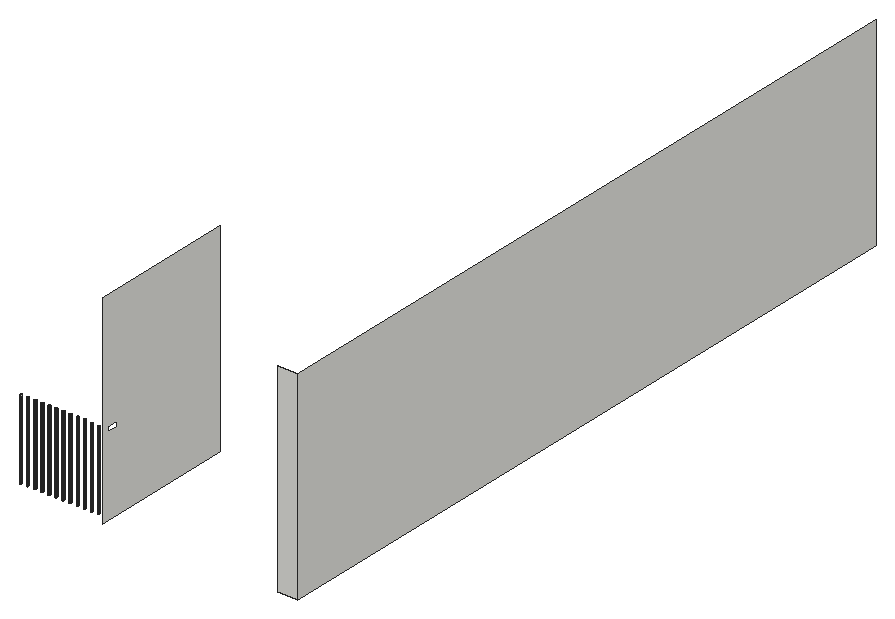
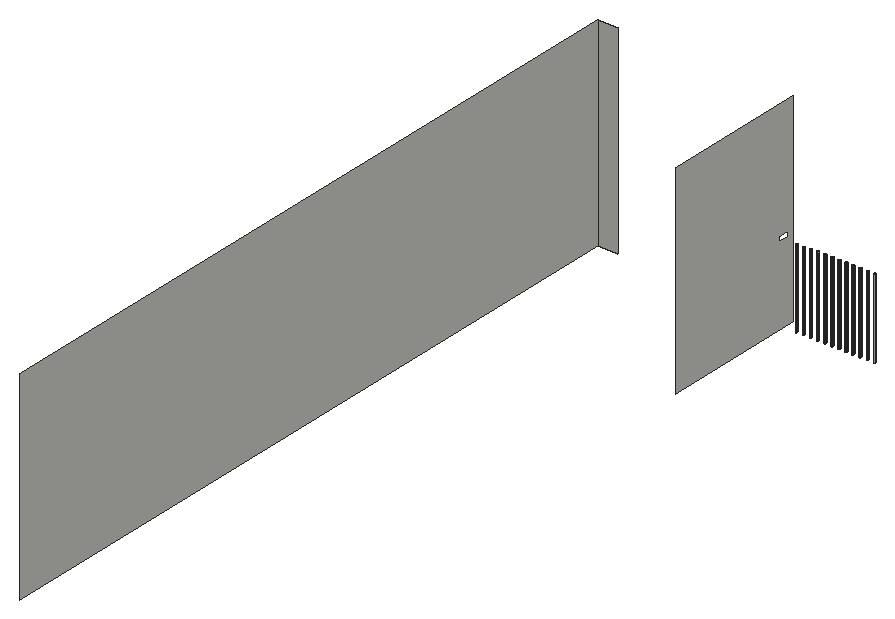
# SketchUp Ruby script. Lengths in inches.
U = 1.inch
M = Sketchup.active_model
def pt(a) = Geom::Point3d.new(a.map { |v| v * U })
def face(e, loops, mat)
  f = e.add_face(loops[0].map { |a| pt(a) })
  loops[1..].each { |l| e.add_face(l.map { |a| pt(a) }).erase! }
  f.material = f.back_material = mat if mat
  f
end
# faces: each face lists its corners as indices into pts; further lists are holes
def faces(e, pts, list, mat = nil) = list.each { |f| face(e, (f[0].is_a?(Array) ? f : [f]).map { |l| l.map { |i| pts[i] } }, mat) }
# xy, xz, yz: faces in a plane at the given z, y or x. An outline is a flat list of corners, or four numbers for a rectangle; further outlines are holes
def ring(l) = l.size == 4 ? [[l[0], l[1]], [l[2], l[1]], [l[2], l[3]], [l[0], l[3]]] : l.each_slice(2).to_a
def flat(e, list, mat, &to3) = list.each { |f| face(e, (f[0].is_a?(Array) ? f : [f]).map { |l| ring(l).map { |u, v| to3.(u, v) } }, mat) }
def xy(e, z, list, mat = nil) = flat(e, list, mat) { |x, y| [x, y, z] }
def xz(e, y, list, mat = nil) = flat(e, list, mat) { |x, z| [x, y, z] }
def yz(e, x, list, mat = nil) = flat(e, list, mat) { |y, z| [x, y, z] }
def lines(e, pts, list) = list.each { |a, b| e.add_line(pt(pts[a]), pt(pts[b])) }
# prism: a flat outline (further loops are holes) pulled along v
def prism(e, loops, v, mat = nil)
  f = face(e, loops, mat); d = Geom::Vector3d.new(v.map { |x| x * U })
  f.pushpull(f.normal.samedirection?(d) ? d.length : -d.length)
end
def box(e, o, s, mat = nil) = prism(e, [[o, [o[0] + s[0], o[1], o[2]], [o[0] + s[0], o[1] + s[1], o[2]], [o[0], o[1] + s[1], o[2]]]], [0, 0, s[2]], mat)
def at(x, y, z, deg = 0) = Geom::Transformation.translation(pt([x, y, z])) * Geom::Transformation.rotation(ORIGIN, Z_AXIS, deg.degrees)
def axes(o, x, y, z) = Geom::Transformation.new([*x, 0, *y, 0, *z, 0, *pt(o).to_a, 1])
def part(name) = M.definitions.add(name)
# library, detail: a bought-in or finely detailed component or shape, given as its bounding box
def library(name, o, s) = part(name).tap { |d| box(d.entities, o, s) }
def detail(e, o, s) = box(e.add_group.entities, o, s)
def put(e, d, t, mat = nil) = e.add_instance(d, t).tap { |i| i.material = mat if mat }
def group(e, t, mat = nil) = e.add_group.tap { |g| g.transformation = t; g.material = mat if mat }.entities
root = M.entities
xy(root,614.8125,[[453.86,132.04,453.64,132.07,453.45,132.15,453.28,132.28,453.15,132.45,453.07,132.64,453.04,132.85,453.07,133.06,453.15,133.26,453.28,133.43,453.45,133.56,453.64,133.64,453.86,133.67,454.07,133.64,454.26,133.56,454.43,133.43,454.56,133.26,454.64,133.06,454.67,132.85,454.64,132.64,454.56,132.45,454.43,132.28,454.26,132.15,454.07,132.07],[459.48,132.04,459.27,132.07,459.07,132.15,458.91,132.28,458.78,132.45,458.7,132.64,458.67,132.85,458.7,133.06,458.78,133.26,458.91,133.43,459.07,133.56,459.27,133.64,459.48,133.67,459.69,133.64,459.89,133.56,460.05,133.43,460.18,133.26,460.27,133.06,460.29,132.85,460.27,132.64,460.18,132.45,460.05,132.28,459.89,132.15,459.69,132.07],[465.54,132.04,465.33,132.07,465.14,132.15,464.97,132.28,464.84,132.45,464.76,132.64,464.73,132.85,464.76,133.06,464.84,133.26,464.97,133.43,465.14,133.56,465.33,133.64,465.54,133.67,465.75,133.64,465.95,133.56,466.12,133.43,466.25,133.26,466.33,133.06,466.36,132.85,466.33,132.64,466.25,132.45,466.12,132.28,465.95,132.15,465.75,132.07],[471.54,132.04,471.33,132.07,471.14,132.15,470.97,132.28,470.84,132.45,470.76,132.64,470.73,132.85,470.76,133.06,470.84,133.26,470.97,133.43,471.14,133.56,471.33,133.64,471.54,133.67,471.75,133.64,471.95,133.56,472.12,133.43,472.25,133.26,472.33,133.06,472.36,132.85,472.33,132.64,472.25,132.45,472.12,132.28,471.95,132.15,471.75,132.07],[477.23,132.04,477.02,132.07,476.82,132.15,476.66,132.28,476.53,132.45,476.45,132.64,476.42,132.85,476.45,133.06,476.53,133.26,476.66,133.43,476.82,133.56,477.02,133.64,477.23,133.67,477.44,133.64,477.64,133.56,477.8,133.43,477.93,133.26,478.02,133.06,478.04,132.85,478.02,132.64,477.93,132.45,477.8,132.28,477.64,132.15,477.44,132.07],
  [483.11,132.04,482.89,132.07,482.7,132.15,482.53,132.28,482.4,132.45,482.32,132.64,482.29,132.85,482.32,133.06,482.4,133.26,482.53,133.43,482.7,133.56,482.89,133.64,483.11,133.67,483.32,133.64,483.51,133.56,483.68,133.43,483.81,133.26,483.89,133.06,483.92,132.85,483.89,132.64,483.81,132.45,483.68,132.28,483.51,132.15,483.32,132.07],[488.98,132.04,488.77,132.07,488.57,132.15,488.41,132.28,488.28,132.45,488.2,132.64,488.17,132.85,488.2,133.06,488.28,133.26,488.41,133.43,488.57,133.56,488.77,133.64,488.98,133.67,489.19,133.64,489.39,133.56,489.55,133.43,489.68,133.26,489.77,133.06,489.79,132.85,489.77,132.64,489.68,132.45,489.55,132.28,489.39,132.15,489.19,132.07],[494.92,132.04,494.71,132.07,494.51,132.15,494.34,132.28,494.21,132.45,494.13,132.64,494.11,132.85,494.13,133.06,494.21,133.26,494.34,133.43,494.51,133.56,494.71,133.64,494.92,133.67,495.13,133.64,495.32,133.56,495.49,133.43,495.62,133.26,495.7,133.06,495.73,132.85,495.7,132.64,495.62,132.45,495.49,132.28,495.32,132.15,495.13,132.07],[500.86,132.04,500.64,132.07,500.45,132.15,500.28,132.28,500.15,132.45,500.07,132.64,500.04,132.85,500.07,133.06,500.15,133.26,500.28,133.43,500.45,133.56,500.64,133.64,500.86,133.67,501.07,133.64,501.26,133.56,501.43,133.43,501.56,133.26,501.64,133.06,501.67,132.85,501.64,132.64,501.56,132.45,501.43,132.28,501.26,132.15,501.07,132.07],[506.67,132.04,506.46,132.07,506.26,132.15,506.09,132.28,505.96,132.45,505.88,132.64,505.86,132.85,505.88,133.06,505.96,133.26,506.09,133.43,506.26,133.56,506.46,133.64,506.67,133.67,506.88,133.64,507.07,133.56,507.24,133.43,507.37,133.26,507.45,133.06,507.48,132.85,507.45,132.64,507.37,132.45,507.24,132.28,507.07,132.15,506.88,132.07],
  [512.54,132.04,512.33,132.07,512.14,132.15,511.97,132.28,511.84,132.45,511.76,132.64,511.73,132.85,511.76,133.06,511.84,133.26,511.97,133.43,512.14,133.56,512.33,133.64,512.54,133.67,512.75,133.64,512.95,133.56,513.12,133.43,513.25,133.26,513.33,133.06,513.36,132.85,513.33,132.64,513.25,132.45,513.12,132.28,512.95,132.15,512.75,132.07],[518.54,132.04,518.33,132.07,518.14,132.15,517.97,132.28,517.84,132.45,517.76,132.64,517.73,132.85,517.76,133.06,517.84,133.26,517.97,133.43,518.14,133.56,518.33,133.64,518.54,133.67,518.75,133.64,518.95,133.56,519.12,133.43,519.25,133.26,519.33,133.06,519.36,132.85,519.33,132.64,519.25,132.45,519.12,132.28,518.95,132.15,518.75,132.07]])
xz(root,124.5,[[673.48,614.8125,690.4375,782.8125]])
yz(root,528.75,[[[124.5,614.8125,246,782.8125],[129.43,680.58,138.74,684.77]]])
yz(root,690.4375,[[124.5,614.8125,724.5,782.8125]])
p = [[453.64,132.07,614.8125],[453.86,132.04,614.8125],[453.86,132.04,680.58],[453.64,132.07,680.58],[454.07,132.07,614.8125],[454.07,132.07,680.58],
  [459.27,132.07,614.8125],[459.48,132.04,614.8125],[459.48,132.04,680.58],[459.27,132.07,680.58],[459.69,132.07,614.8125],[459.69,132.07,680.58],
  [465.33,132.07,614.8125],[465.54,132.04,614.8125],[465.54,132.04,680.58],[465.33,132.07,680.58],[465.75,132.07,614.8125],[465.75,132.07,680.58],
  [471.33,132.07,614.8125],[471.54,132.04,614.8125],[471.54,132.04,680.58],[471.33,132.07,680.58],[471.75,132.07,614.8125],[471.75,132.07,680.58],
  [477.02,132.07,614.8125],[477.23,132.04,614.8125],[477.23,132.04,680.58],[477.02,132.07,680.58],[477.44,132.07,614.8125],[477.44,132.07,680.58],
  [482.89,132.07,614.8125],[483.11,132.04,614.8125],[483.11,132.04,680.58],[482.89,132.07,680.58],[483.32,132.07,614.8125],[483.32,132.07,680.58],
  [488.77,132.07,614.8125],[488.98,132.04,614.8125],[488.98,132.04,680.58],[488.77,132.07,680.58],[489.19,132.07,614.8125],[489.19,132.07,680.58],
  [494.71,132.07,614.8125],[494.92,132.04,614.8125],[494.92,132.04,680.58],[494.71,132.07,680.58],[495.13,132.07,614.8125],[495.13,132.07,680.58],
  [500.64,132.07,614.8125],[500.86,132.04,614.8125],[500.86,132.04,680.58],[500.64,132.07,680.58],[501.07,132.07,614.8125],[501.07,132.07,680.58],
  [506.46,132.07,614.8125],[506.67,132.04,614.8125],[506.67,132.04,680.58],[506.46,132.07,680.58],[506.88,132.07,614.8125],[506.88,132.07,680.58],
  [512.33,132.07,614.8125],[512.54,132.04,614.8125],[512.54,132.04,679.96],[512.33,132.07,679.96],[512.75,132.07,614.8125],[512.75,132.07,679.96],
  [518.33,132.07,614.8125],[518.54,132.04,614.8125],[518.54,132.04,679.96],[518.33,132.07,679.96],[518.75,132.07,614.8125],[518.75,132.07,679.96],
  [453.45,132.15,614.8125],[453.45,132.15,680.58],[454.26,132.15,614.8125],[454.26,132.15,680.58],[459.07,132.15,614.8125],[459.07,132.15,680.58],
  [459.89,132.15,614.8125],[459.89,132.15,680.58],[465.14,132.15,614.8125],[465.14,132.15,680.58],[465.95,132.15,614.8125],[465.95,132.15,680.58],
  [471.14,132.15,614.8125],[471.14,132.15,680.58],[471.95,132.15,614.8125],[471.95,132.15,680.58],[476.82,132.15,614.8125],[476.82,132.15,680.58],
  [477.64,132.15,614.8125],[477.64,132.15,680.58],[482.7,132.15,614.8125],[482.7,132.15,680.58],[483.51,132.15,614.8125],[483.51,132.15,680.58],
  [488.57,132.15,614.8125],[488.57,132.15,680.58],[489.39,132.15,614.8125],[489.39,132.15,680.58],[494.51,132.15,614.8125],[494.51,132.15,680.58],
  [495.32,132.15,614.8125],[495.32,132.15,680.58],[500.45,132.15,614.8125],[500.45,132.15,680.58],[501.26,132.15,614.8125],[501.26,132.15,680.58],
  [506.26,132.15,614.8125],[506.26,132.15,680.58],[507.07,132.15,614.8125],[507.07,132.15,680.58],[512.14,132.15,614.8125],[512.14,132.15,679.96],
  [512.95,132.15,614.8125],[512.95,132.15,679.96],[518.14,132.15,614.8125],[518.14,132.15,679.96],[518.95,132.15,614.8125],[518.95,132.15,679.96],
  [454.43,132.28,614.8125],[454.43,132.28,680.58],[458.91,132.28,614.8125],[458.91,132.28,680.58],[460.05,132.28,614.8125],[460.05,132.28,680.58],
  [464.97,132.28,614.8125],[464.97,132.28,680.58],[466.12,132.28,614.8125],[466.12,132.28,680.58],[470.97,132.28,614.8125],[470.97,132.28,680.58],
  [472.12,132.28,614.8125],[472.12,132.28,680.58],[476.66,132.28,614.8125],[476.66,132.28,680.58],[477.8,132.28,614.8125],[477.8,132.28,680.58],
  [482.53,132.28,614.8125],[482.53,132.28,680.58],[483.68,132.28,614.8125],[483.68,132.28,680.58],[488.41,132.28,614.8125],[488.41,132.28,680.58],
  [489.55,132.28,614.8125],[489.55,132.28,680.58],[494.34,132.28,614.8125],[494.34,132.28,680.58],[495.49,132.28,614.8125],[495.49,132.28,680.58],
  [500.28,132.28,614.8125],[500.28,132.28,680.58],[501.43,132.28,614.8125],[501.43,132.28,680.58],[506.09,132.28,614.8125],[506.09,132.28,680.58],
  [507.24,132.28,614.8125],[507.24,132.28,680.58],[511.97,132.28,614.8125],[511.97,132.28,679.96],[513.12,132.28,614.8125],[513.12,132.28,679.96],
  [517.97,132.28,614.8125],[517.97,132.28,679.96],[519.12,132.28,614.8125],[519.12,132.28,679.96],[454.56,132.45,614.8125],[454.56,132.45,680.58],
  [458.78,132.45,614.8125],[458.78,132.45,680.58],[460.18,132.45,614.8125],[460.18,132.45,680.58],[464.84,132.45,614.8125],[464.84,132.45,680.58],
  [466.25,132.45,614.8125],[466.25,132.45,680.58],[470.84,132.45,614.8125],[470.84,132.45,680.58],[472.25,132.45,614.8125],[472.25,132.45,680.58],
  [476.53,132.45,614.8125],[476.53,132.45,680.58],[477.93,132.45,614.8125],[477.93,132.45,680.58],[482.4,132.45,614.8125],[482.4,132.45,680.58],
  [483.81,132.45,614.8125],[483.81,132.45,680.58],[488.28,132.45,614.8125],[488.28,132.45,680.58],[489.68,132.45,614.8125],[489.68,132.45,680.58],
  [494.21,132.45,614.8125],[494.21,132.45,680.58],[495.62,132.45,614.8125],[495.62,132.45,680.58],[500.15,132.45,614.8125],[500.15,132.45,680.58],
  [501.56,132.45,614.8125],[501.56,132.45,680.58],[505.96,132.45,614.8125],[505.96,132.45,680.58],[507.37,132.45,614.8125],[507.37,132.45,680.58],
  [511.84,132.45,614.8125],[511.84,132.45,679.96],[513.25,132.45,614.8125],[513.25,132.45,679.96],[517.84,132.45,614.8125],[517.84,132.45,679.96],
  [519.25,132.45,614.8125],[519.25,132.45,679.96],[454.64,132.64,614.8125],[454.64,132.64,680.58],[458.7,132.64,614.8125],[458.7,132.64,680.58],
  [460.27,132.64,614.8125],[460.27,132.64,680.58],[464.76,132.64,614.8125],[464.76,132.64,680.58],[466.33,132.64,614.8125],[466.33,132.64,680.58],
  [470.76,132.64,614.8125],[470.76,132.64,680.58],[472.33,132.64,614.8125],[472.33,132.64,680.58],[476.45,132.64,614.8125],[476.45,132.64,680.58],
  [478.02,132.64,614.8125],[478.02,132.64,680.58],[482.32,132.64,614.8125],[482.32,132.64,680.58],[483.89,132.64,614.8125],[483.89,132.64,680.58],
  [488.2,132.64,614.8125],[488.2,132.64,680.58],[489.77,132.64,614.8125],[489.77,132.64,680.58],[494.13,132.64,614.8125],[494.13,132.64,680.58],
  [495.7,132.64,614.8125],[495.7,132.64,680.58],[500.07,132.64,614.8125],[500.07,132.64,680.58],[501.64,132.64,614.8125],[501.64,132.64,680.58],
  [505.88,132.64,614.8125],[505.88,132.64,680.58],[507.45,132.64,614.8125],[507.45,132.64,680.58],[511.76,132.64,614.8125],[511.76,132.64,679.96],
  [513.33,132.64,614.8125],[513.33,132.64,679.96],[517.76,132.64,614.8125],[517.76,132.64,679.96],[519.33,132.64,614.8125],[519.33,132.64,679.96],
  [454.67,132.85,614.8125],[454.67,132.85,680.58],[458.67,132.85,614.8125],[458.67,132.85,680.58],[460.29,132.85,614.8125],[460.29,132.85,680.58],
  [464.73,132.85,614.8125],[464.73,132.85,680.58],[466.36,132.85,614.8125],[466.36,132.85,680.58],[470.73,132.85,614.8125],[470.73,132.85,680.58],
  [472.36,132.85,614.8125],[472.36,132.85,680.58],[476.42,132.85,614.8125],[476.42,132.85,680.58],[478.04,132.85,614.8125],[478.04,132.85,680.58],
  [482.29,132.85,614.8125],[482.29,132.85,680.58],[483.92,132.85,614.8125],[483.92,132.85,680.58],[488.17,132.85,614.8125],[488.17,132.85,680.58],
  [489.79,132.85,614.8125],[489.79,132.85,680.58],[494.11,132.85,614.8125],[494.11,132.85,680.58],[495.73,132.85,614.8125],[495.73,132.85,680.58],
  [500.04,132.85,614.8125],[500.04,132.85,680.58],[501.67,132.85,614.8125],[501.67,132.85,680.58],[505.86,132.85,614.8125],[505.86,132.85,680.58],
  [507.48,132.85,614.8125],[507.48,132.85,680.58],[511.73,132.85,614.8125],[511.73,132.85,679.96],[513.36,132.85,614.8125],[513.36,132.85,679.96],
  [517.73,132.85,614.8125],[517.73,132.85,679.96],[519.36,132.85,614.8125],[519.36,132.85,679.96],[454.64,133.06,614.8125],[454.64,133.06,680.58],
  [458.7,133.06,614.8125],[458.7,133.06,680.58],[460.27,133.06,614.8125],[460.27,133.06,680.58],[464.76,133.06,614.8125],[464.76,133.06,680.58],
  [466.33,133.06,614.8125],[466.33,133.06,680.58],[470.76,133.06,614.8125],[470.76,133.06,680.58],[472.33,133.06,614.8125],[472.33,133.06,680.58],
  [476.45,133.06,614.8125],[476.45,133.06,680.58],[478.02,133.06,614.8125],[478.02,133.06,680.58],[482.32,133.06,614.8125],[482.32,133.06,680.58],
  [483.89,133.06,614.8125],[483.89,133.06,680.58],[488.2,133.06,614.8125],[488.2,133.06,680.58],[489.77,133.06,614.8125],[489.77,133.06,680.58],
  [494.13,133.06,614.8125],[494.13,133.06,680.58],[495.7,133.06,614.8125],[495.7,133.06,680.58],[500.07,133.06,614.8125],[500.07,133.06,680.58],
  [501.64,133.06,614.8125],[501.64,133.06,680.58],[505.88,133.06,614.8125],[505.88,133.06,680.58],[507.45,133.06,614.8125],[507.45,133.06,680.58],
  [511.76,133.06,614.8125],[511.76,133.06,679.96],[513.33,133.06,614.8125],[513.33,133.06,679.96],[517.76,133.06,614.8125],[517.76,133.06,679.96],
  [519.33,133.06,614.8125],[519.33,133.06,679.96],[454.56,133.26,614.8125],[454.56,133.26,680.58],[458.78,133.26,614.8125],[458.78,133.26,680.58],
  [460.18,133.26,614.8125],[460.18,133.26,680.58],[464.84,133.26,614.8125],[464.84,133.26,680.58],[466.25,133.26,614.8125],[466.25,133.26,680.58],
  [470.84,133.26,614.8125],[470.84,133.26,680.58],[472.25,133.26,614.8125],[472.25,133.26,680.58],[476.53,133.26,614.8125],[476.53,133.26,680.58],
  [477.93,133.26,614.8125],[477.93,133.26,680.58],[482.4,133.26,614.8125],[482.4,133.26,680.58],[483.81,133.26,614.8125],[483.81,133.26,680.58],
  [488.28,133.26,614.8125],[488.28,133.26,680.58],[489.68,133.26,614.8125],[489.68,133.26,680.58],[494.21,133.26,614.8125],[494.21,133.26,680.58],
  [495.62,133.26,614.8125],[495.62,133.26,680.58],[500.15,133.26,614.8125],[500.15,133.26,680.58],[501.56,133.26,614.8125],[501.56,133.26,680.58],
  [505.96,133.26,614.8125],[505.96,133.26,680.58],[507.37,133.26,614.8125],[507.37,133.26,680.58],[511.84,133.26,614.8125],[511.84,133.26,679.96],
  [513.25,133.26,614.8125],[513.25,133.26,679.96],[517.84,133.26,614.8125],[517.84,133.26,679.96],[519.25,133.26,614.8125],[519.25,133.26,679.96],
  [454.43,133.43,614.8125],[454.43,133.43,680.58],[458.91,133.43,614.8125],[458.91,133.43,680.58],[460.05,133.43,614.8125],[460.05,133.43,680.58],
  [464.97,133.43,614.8125],[464.97,133.43,680.58],[466.12,133.43,614.8125],[466.12,133.43,680.58],[470.97,133.43,614.8125],[470.97,133.43,680.58],
  [472.12,133.43,614.8125],[472.12,133.43,680.58],[476.66,133.43,614.8125],[476.66,133.43,680.58],[477.8,133.43,614.8125],[477.8,133.43,680.58],
  [482.53,133.43,614.8125],[482.53,133.43,680.58],[483.68,133.43,614.8125],[483.68,133.43,680.58],[488.41,133.43,614.8125],[488.41,133.43,680.58],
  [489.55,133.43,614.8125],[489.55,133.43,680.58],[494.34,133.43,614.8125],[494.34,133.43,680.58],[495.49,133.43,614.8125],[495.49,133.43,680.58],
  [500.28,133.43,614.8125],[500.28,133.43,680.58],[501.43,133.43,614.8125],[501.43,133.43,680.58],[506.09,133.43,614.8125],[506.09,133.43,680.58],
  [507.24,133.43,614.8125],[507.24,133.43,680.58],[511.97,133.43,614.8125],[511.97,133.43,679.96],[513.12,133.43,614.8125],[513.12,133.43,679.96],
  [517.97,133.43,614.8125],[517.97,133.43,679.96],[519.12,133.43,614.8125],[519.12,133.43,679.96],[454.26,133.56,614.8125],[454.26,133.56,680.58],
  [459.07,133.56,614.8125],[459.07,133.56,680.58],[459.89,133.56,614.8125],[459.89,133.56,680.58],[465.14,133.56,614.8125],[465.14,133.56,680.58],
  [465.95,133.56,614.8125],[465.95,133.56,680.58],[471.14,133.56,614.8125],[471.14,133.56,680.58],[471.95,133.56,614.8125],[471.95,133.56,680.58],
  [476.82,133.56,614.8125],[476.82,133.56,680.58],[477.64,133.56,614.8125],[477.64,133.56,680.58],[482.7,133.56,614.8125],[482.7,133.56,680.58],
  [483.51,133.56,614.8125],[483.51,133.56,680.58],[488.57,133.56,614.8125],[488.57,133.56,680.58],[489.39,133.56,614.8125],[489.39,133.56,680.58],
  [494.51,133.56,614.8125],[494.51,133.56,680.58],[495.32,133.56,614.8125],[495.32,133.56,680.58],[500.45,133.56,614.8125],[500.45,133.56,680.58],
  [501.26,133.56,614.8125],[501.26,133.56,680.58],[506.26,133.56,614.8125],[506.26,133.56,680.58],[507.07,133.56,614.8125],[507.07,133.56,680.58],
  [512.14,133.56,614.8125],[512.14,133.56,679.96],[512.95,133.56,614.8125],[512.95,133.56,679.96],[518.14,133.56,614.8125],[518.14,133.56,679.96],
  [518.95,133.56,614.8125],[518.95,133.56,679.96],[453.64,133.64,614.8125],[453.45,133.56,614.8125],[453.45,133.56,680.58],[453.64,133.64,680.58],
  [453.86,133.67,614.8125],[453.86,133.67,680.58],[454.07,133.64,614.8125],[454.07,133.64,680.58],[459.27,133.64,614.8125],[459.27,133.64,680.58],
  [459.48,133.67,614.8125],[459.48,133.67,680.58],[459.69,133.64,614.8125],[459.69,133.64,680.58],[465.33,133.64,614.8125],[465.33,133.64,680.58],
  [465.54,133.67,614.8125],[465.54,133.67,680.58],[465.75,133.64,614.8125],[465.75,133.64,680.58],[471.33,133.64,614.8125],[471.33,133.64,680.58],
  [471.54,133.67,614.8125],[471.54,133.67,680.58],[471.75,133.64,614.8125],[471.75,133.64,680.58],[477.02,133.64,614.8125],[477.02,133.64,680.58],
  [477.23,133.67,614.8125],[477.23,133.67,680.58],[477.44,133.64,614.8125],[477.44,133.64,680.58],[482.89,133.64,614.8125],[482.89,133.64,680.58],
  [483.11,133.67,614.8125],[483.11,133.67,680.58],[483.32,133.64,614.8125],[483.32,133.64,680.58],[488.77,133.64,614.8125],[488.77,133.64,680.58],
  [488.98,133.67,614.8125],[488.98,133.67,680.58],[489.19,133.64,614.8125],[489.19,133.64,680.58],[494.71,133.64,614.8125],[494.71,133.64,680.58],
  [494.92,133.67,614.8125],[494.92,133.67,680.58],[495.13,133.64,614.8125],[495.13,133.64,680.58],[500.64,133.64,614.8125],[500.64,133.64,680.58],
  [500.86,133.67,614.8125],[500.86,133.67,680.58],[501.07,133.64,614.8125],[501.07,133.64,680.58],[506.46,133.64,614.8125],[506.46,133.64,680.58],
  [506.67,133.67,614.8125],[506.67,133.67,680.58],[506.88,133.64,614.8125],[506.88,133.64,680.58],[512.33,133.64,614.8125],[512.33,133.64,679.96],
  [512.54,133.67,614.8125],[512.54,133.67,679.96],[512.75,133.64,614.8125],[512.75,133.64,679.96],[518.33,133.64,614.8125],[518.33,133.64,679.96],
  [518.54,133.67,614.8125],[518.54,133.67,679.96],[518.75,133.64,614.8125],[518.75,133.64,679.96],[518.38,132.57,680.58],[518.38,132.57,614.8125],
  [512.51,132.57,680.58],[512.51,132.57,614.8125],[506.63,132.57,680.58],[506.63,132.57,614.8125],[500.76,132.57,680.58],[500.76,132.57,614.8125],
  [494.88,132.57,680.58],[494.88,132.57,614.8125],[489.01,132.57,680.58],[489.01,132.57,614.8125],[483.13,132.57,680.58],[483.13,132.57,614.8125],
  [477.26,132.57,680.58],[477.26,132.57,614.8125],[471.38,132.57,680.58],[471.38,132.57,614.8125],[465.51,132.57,680.58],[465.51,132.57,614.8125],
  [459.63,132.57,680.58],[459.63,132.57,614.8125],[453.76,132.57,680.58],[453.76,132.57,614.8125]]
faces(root,p,[[0,1,2,3],[1,4,5,2],[6,7,8,9],[7,10,11,8],[12,13,14,15],[13,16,17,14],[18,19,20,21],[19,22,23,20],
  [24,25,26,27],[25,28,29,26],[30,31,32,33],[31,34,35,32],[36,37,38,39],[37,40,41,38],[42,43,44,45],[43,46,47,44],
  [48,49,50,51],[49,52,53,50],[54,55,56,57],[55,58,59,56],[60,61,62,63],[61,64,65,62],[66,67,68,69],[67,70,71,68],
  [72,0,3,73],[4,74,75,5],[76,6,9,77],[10,78,79,11],[80,12,15,81],[16,82,83,17],[84,18,21,85],[22,86,87,23],
  [88,24,27,89],[28,90,91,29],[92,30,33,93],[34,94,95,35],[96,36,39,97],[40,98,99,41],[100,42,45,101],[46,102,103,47],
  [104,48,51,105],[52,106,107,53],[108,54,57,109],[58,110,111,59],[112,60,63,113],[64,114,115,65],[116,66,69,117],[70,118,119,71],
  [74,120,121,75],[122,76,77,123],[78,124,125,79],[126,80,81,127],[82,128,129,83],[130,84,85,131],[86,132,133,87],[134,88,89,135],
  [90,136,137,91],[138,92,93,139],[94,140,141,95],[142,96,97,143],[98,144,145,99],[146,100,101,147],[102,148,149,103],[150,104,105,151],
  [106,152,153,107],[154,108,109,155],[110,156,157,111],[158,112,113,159],[114,160,161,115],[162,116,117,163],[118,164,165,119],[120,166,167,121],
  [168,122,123,169],[124,170,171,125],[172,126,127,173],[128,174,175,129],[176,130,131,177],[132,178,179,133],[180,134,135,181],[136,182,183,137],
  [184,138,139,185],[140,186,187,141],[188,142,143,189],[144,190,191,145],[192,146,147,193],[148,194,195,149],[196,150,151,197],[152,198,199,153],
  [200,154,155,201],[156,202,203,157],[204,158,159,205],[160,206,207,161],[208,162,163,209],[164,210,211,165],[166,212,213,167],[214,168,169,215],
  [170,216,217,171],[218,172,173,219],[174,220,221,175],[222,176,177,223],[178,224,225,179],[226,180,181,227],[182,228,229,183],[230,184,185,231],
  [186,232,233,187],[234,188,189,235],[190,236,237,191],[238,192,193,239],[194,240,241,195],[242,196,197,243],[198,244,245,199],[246,200,201,247],
  [202,248,249,203],[250,204,205,251],[206,252,253,207],[254,208,209,255],[210,256,257,211],[212,258,259,213],[260,214,215,261],[216,262,263,217],
  [264,218,219,265],[220,266,267,221],[268,222,223,269],[224,270,271,225],[272,226,227,273],[228,274,275,229],[276,230,231,277],[232,278,279,233],
  [280,234,235,281],[236,282,283,237],[284,238,239,285],[240,286,287,241],[288,242,243,289],[244,290,291,245],[292,246,247,293],[248,294,295,249],
  [296,250,251,297],[252,298,299,253],[300,254,255,301],[256,302,303,257],[258,304,305,259],[306,260,261,307],[262,308,309,263],[310,264,265,311],
  [266,312,313,267],[314,268,269,315],[270,316,317,271],[318,272,273,319],[274,320,321,275],[322,276,277,323],[278,324,325,279],[326,280,281,327],
  [282,328,329,283],[330,284,285,331],[286,332,333,287],[334,288,289,335],[290,336,337,291],[338,292,293,339],[294,340,341,295],[342,296,297,343],
  [298,344,345,299],[346,300,301,347],[302,348,349,303],[304,350,351,305],[352,306,307,353],[308,354,355,309],[356,310,311,357],[312,358,359,313],
  [360,314,315,361],[316,362,363,317],[364,318,319,365],[320,366,367,321],[368,322,323,369],[324,370,371,325],[372,326,327,373],[328,374,375,329],
  [376,330,331,377],[332,378,379,333],[380,334,335,381],[336,382,383,337],[384,338,339,385],[340,386,387,341],[388,342,343,389],[344,390,391,345],
  [392,346,347,393],[348,394,395,349],[350,396,397,351],[398,352,353,399],[354,400,401,355],[402,356,357,403],[358,404,405,359],[406,360,361,407],
  [362,408,409,363],[410,364,365,411],[366,412,413,367],[414,368,369,415],[370,416,417,371],[418,372,373,419],[374,420,421,375],[422,376,377,423],
  [378,424,425,379],[426,380,381,427],[382,428,429,383],[430,384,385,431],[386,432,433,387],[434,388,389,435],[390,436,437,391],[438,392,393,439],
  [394,440,441,395],[396,442,443,397],[444,398,399,445],[400,446,447,401],[448,402,403,449],[404,450,451,405],[452,406,407,453],[408,454,455,409],
  [456,410,411,457],[412,458,459,413],[460,414,415,461],[416,462,463,417],[464,418,419,465],[420,466,467,421],[468,422,423,469],[424,470,471,425],
  [472,426,427,473],[428,474,475,429],[476,430,431,477],[432,478,479,433],[480,434,435,481],[436,482,483,437],[484,438,439,485],[440,486,487,441],
  [488,489,490,491],[492,488,491,493],[494,492,493,495],[442,494,495,443],[496,444,445,497],[498,496,497,499],[500,498,499,501],[446,500,501,447],
  [502,448,449,503],[504,502,503,505],[506,504,505,507],[450,506,507,451],[508,452,453,509],[510,508,509,511],[512,510,511,513],[454,512,513,455],
  [514,456,457,515],[516,514,515,517],[518,516,517,519],[458,518,519,459],[520,460,461,521],[522,520,521,523],[524,522,523,525],[462,524,525,463],
  [526,464,465,527],[528,526,527,529],[530,528,529,531],[466,530,531,467],[532,468,469,533],[534,532,533,535],[536,534,535,537],[470,536,537,471],
  [538,472,473,539],[540,538,539,541],[542,540,541,543],[474,542,543,475],[544,476,477,545],[546,544,545,547],[548,546,547,549],[478,548,549,479],
  [550,480,481,551],[552,550,551,553],[554,552,553,555],[482,554,555,483],[556,484,485,557],[558,556,557,559],[560,558,559,561],[486,560,561,487]])
lines(root,p,[[562,563],[564,565],[566,567],[568,569],[570,571],[572,573],[574,575],[576,577],[578,579],[580,581],[582,583],[584,585]])
